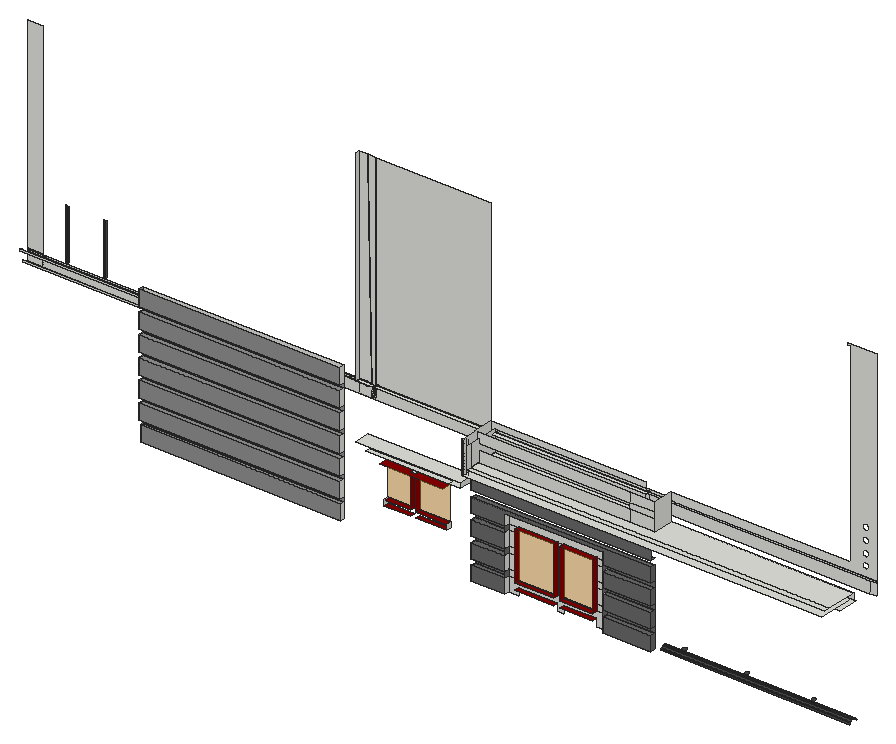
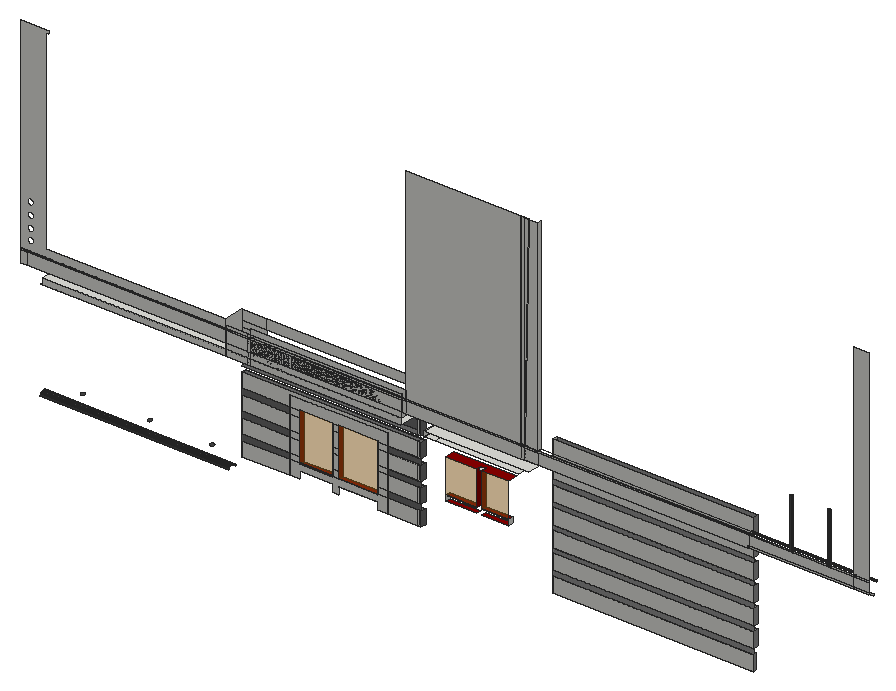
# SketchUp Ruby script. Lengths in inches.
U = 1.inch
M = Sketchup.active_model
def pt(a) = Geom::Point3d.new(a.map { |v| v * U })
def face(e, loops, mat)
  f = e.add_face(loops[0].map { |a| pt(a) })
  loops[1..].each { |l| e.add_face(l.map { |a| pt(a) }).erase! }
  f.material = f.back_material = mat if mat
  f
end
# faces: each face lists its corners as indices into pts; further lists are holes
def faces(e, pts, list, mat = nil) = list.each { |f| face(e, (f[0].is_a?(Array) ? f : [f]).map { |l| l.map { |i| pts[i] } }, mat) }
# xy, xz, yz: faces in a plane at the given z, y or x. An outline is a flat list of corners, or four numbers for a rectangle; further outlines are holes
def ring(l) = l.size == 4 ? [[l[0], l[1]], [l[2], l[1]], [l[2], l[3]], [l[0], l[3]]] : l.each_slice(2).to_a
def flat(e, list, mat, &to3) = list.each { |f| face(e, (f[0].is_a?(Array) ? f : [f]).map { |l| ring(l).map { |u, v| to3.(u, v) } }, mat) }
def xy(e, z, list, mat = nil) = flat(e, list, mat) { |x, y| [x, y, z] }
def xz(e, y, list, mat = nil) = flat(e, list, mat) { |x, z| [x, y, z] }
def yz(e, x, list, mat = nil) = flat(e, list, mat) { |y, z| [x, y, z] }
def lines(e, pts, list) = list.each { |a, b| e.add_line(pt(pts[a]), pt(pts[b])) }
# prism: a flat outline (further loops are holes) pulled along v
def prism(e, loops, v, mat = nil)
  f = face(e, loops, mat); d = Geom::Vector3d.new(v.map { |x| x * U })
  f.pushpull(f.normal.samedirection?(d) ? d.length : -d.length)
end
def box(e, o, s, mat = nil) = prism(e, [[o, [o[0] + s[0], o[1], o[2]], [o[0] + s[0], o[1] + s[1], o[2]], [o[0], o[1] + s[1], o[2]]]], [0, 0, s[2]], mat)
def at(x, y, z, deg = 0) = Geom::Transformation.translation(pt([x, y, z])) * Geom::Transformation.rotation(ORIGIN, Z_AXIS, deg.degrees)
def axes(o, x, y, z) = Geom::Transformation.new([*x, 0, *y, 0, *z, 0, *pt(o).to_a, 1])
def part(name) = M.definitions.add(name)
# library, detail: a bought-in or finely detailed component or shape, given as its bounding box
def library(name, o, s) = part(name).tap { |d| box(d.entities, o, s) }
def detail(e, o, s) = box(e.add_group.entities, o, s)
def put(e, d, t, mat = nil) = e.add_instance(d, t).tap { |i| i.material = mat if mat }
def group(e, t, mat = nil) = e.add_group.tap { |g| g.transformation = t; g.material = mat if mat }.entities
root = M.entities
M.materials.add("[0021_DarkRed]").color = [139, 0, 0]
M.materials.add("[0134_DimGray]").color = [105, 105, 105]
M.materials.add("[0137_Black]").color = [71, 71, 71]
M.materials.add("[Color M05]").color = [145, 145, 145]
M.materials.add("[Translucent Glass Gray]").color = [191, 123, 24]
M.materials["[Translucent Glass Gray]"].alpha = 0.5
xy(root,168.55,[[82.85,16.375,200.79,18.1875]])
xy(root,170.27,[[284.66,7.0625,304.13,10.0625],[362.13,7.0625,390.0625,10.0625]],"[0134_DimGray]")
xy(root,173.53,[[404.27,13.19,404.56,13.23,404.83,13.34,405.0625,13.52,405.24,13.76,405.35,14.03,405.39,14.32,405.35,14.61,405.24,14.88,405.0625,15.11,404.83,15.29,404.56,15.41,404.27,15.44,403.97,15.41,403.7,15.29,403.47,15.11,403.29,14.88,403.18,14.61,403.14,14.32,403.18,14.03,403.29,13.76,403.47,13.52,403.7,13.34,403.97,13.23],[440.77,13.19,441.06,13.23,441.33,13.34,441.5625,13.52,441.74,13.76,441.85,14.03,441.89,14.32,441.85,14.61,441.74,14.88,441.5625,15.11,441.33,15.29,441.06,15.41,440.77,15.44,440.47,15.41,440.2,15.29,439.97,15.11,439.79,14.88,439.68,14.61,439.64,14.32,439.68,14.03,439.79,13.76,439.97,13.52,440.2,13.34,440.47,13.23],[480.14,13.19,480.43,13.23,480.7,13.34,480.9375,13.52,481.12,13.76,481.23,14.03,481.27,14.32,481.23,14.61,481.12,14.88,480.9375,15.11,480.7,15.29,480.43,15.41,480.14,15.44,479.85,15.41,479.58,15.29,479.35,15.11,479.17,14.88,479.05,14.61,479.02,14.32,479.05,14.03,479.17,13.76,479.35,13.52,479.58,13.34,479.85,13.23]],"[0137_Black]")
xy(root,174.59,[[310.13,7.0625,333.13,10.0625],[336.9,7.0625,356.13,10.0625]],"[0021_DarkRed]")
xy(root,177.65,[[82.85,16.375,200.79,18.1875]],"[Color M05]")
xy(root,178.32,[[310.13,7.0625,333.13,10.0625],[336.9,7.0625,356.13,10.0625]],"[0021_DarkRed]")
xy(root,178.6875,[[284.66,7.0625,304.13,10.0625],[362.13,7.0625,390.0625,10.0625]],"[0134_DimGray]")
xy(root,180.55,[[82.85,15.1875,200.79,18.1875]])
xy(root,182.27,[[284.66,7.0625,304.13,10.0625],[362.13,7.0625,390.0625,10.0625]],"[0134_DimGray]")
xy(root,189.65,[[82.85,15.1875,200.79,18.1875]],"[Color M05]")
xy(root,190.54,[[231.66,9.1875,247.4,12.1875],[250.1,9.1875,268.54,12.1875]],"[0021_DarkRed]")
xy(root,190.6875,[[284.66,7.0625,304.13,10.0625],[362.13,7.0625,390.0625,10.0625]],"[0134_DimGray]")
xy(root,192.55,[[82.85,15.1875,200.79,18.1875]])
xy(root,193.6,[[231.66,9.1875,247.4,12.1875],[250.1,9.1875,268.54,12.1875]],"[0021_DarkRed]")
xy(root,194.27,[[284.66,7.0625,304.13,10.0625],[362.13,7.0625,390.0625,10.0625]],"[0134_DimGray]")
xy(root,201.65,[[82.85,15.1875,200.79,18.1875]],"[Color M05]")
xy(root,202.6875,[[284.66,7.0625,304.13,10.0625],[362.13,7.0625,390.0625,10.0625]],"[0134_DimGray]")
xy(root,204.55,[[82.85,15.1875,200.79,18.1875]])
xy(root,206.27,[[284.66,7.0625,304.13,10.0625],[362.13,7.0625,390.0625,10.0625]],"[0134_DimGray]")
xy(root,206.79,[[310.13,7.0625,333.13,10.0625],[336.9,7.0625,356.13,10.0625]],"[0021_DarkRed]")
xy(root,212.79,[[304.13,7.0625,362.13,10.0625]])
xy(root,213.65,[[82.85,15.1875,200.79,18.1875]],"[Color M05]")
xy(root,213.83,[[247.4,9.1875,250.1,12.1875]])
xy(root,213.83,[[231.66,6.1875,231.66,12.1875,247.4,12.1875,247.4,9.1875,250.1,9.1875,250.1,12.1875,268.54,12.1875,268.54,6.1875]],"[0021_DarkRed]")
xy(root,214.6875,[[284.66,7.0625,286.99,10.0625],[286.99,7.0625,390.0625,10.0625]],"[0134_DimGray]")
xy(root,216.55,[[82.85,15.1875,200.79,18.1875]])
xy(root,218.27,[[284.66,7.0625,390.0625,10.0625]],"[0134_DimGray]")
xy(root,219.83,[[225.66,3.1875,274.54,6.1875],[274.54,3.1875,281.16,12.1875],[281.16,3.1875,281.47,12.1875],[225.66,6.1875,274.54,12.1875]])
xy(root,222.71,[[219.91,3.1875,281.47,12.1875]])
xy(root,225.65,[[82.85,15.1875,200.79,18.1875]],"[Color M05]")
xy(root,226.6875,[[335.53,7.0625,375.29,10.0625],[375.29,7.0625,390.0625,10.0625]])
xy(root,226.6875,[[284.66,7.0625,335.53,10.0625]],"[0134_DimGray]")
xy(root,228.47,[[284.05,1.0625,284.41,1.5],[284.41,1.0625,284.41,10.0625,390.0625,10.0625,390.0625,22.0625,495.71,22.0625,495.71,1.0625],[284.41,10.0625,284.66,13.0625],[286.99,10.0625,334.1,22.0625],[334.1,10.0625,375.29,22.0625],
  [375.29,10.0625,390.0625,22.0625],[495.71,10.0625,498.65,22.0625]])
xy(root,228.55,[[82.85,15.1875,200.79,18.1875]])
xy(root,232.22,[[286.99,1.0625,497.29,4.0625],[286.52,4.0625,286.99,22.0625],[286.99,4.0625,497.29,22.0625]])
xy(root,237.65,[[82.85,15.1875,200.79,18.1875]],"[Color M05]")
xy(root,240.55,[[82.85,15.1875,200.79,18.1875]])
xy(root,243,[[206.66,19.6875,214.3,19.75],[206.66,19.75,214.3,22.0625],[214.3,19.75,216.79,21.8125],[216.79,19.75,284.41,22.0625],[284.41,19.75,376.99,22.0625],
  [214.3,21.8125,216.79,22.0625]])
xz(root,1.5,[[284.05,228.47,284.41,247.33]])
xz(root,7.0625,[[284.66,170.27,304.13,178.6875],[362.13,170.27,390.0625,178.6875],[284.66,182.27,304.13,190.6875],[362.13,182.27,390.0625,190.6875],[284.66,194.27,304.13,202.6875],
  [362.13,194.27,390.0625,202.6875],[284.66,206.27,304.13,206.27,304.13,212.79,362.13,212.79,362.13,206.27,390.0625,206.27,390.0625,214.6875,284.66,214.6875],[284.66,218.27,390.0625,226.6875]],"[0134_DimGray]")
xz(root,10.0625,[[284.66,170.27,286.17,178.6875],[286.17,170.27,286.99,178.6875],[286.99,170.27,304.13,178.6875],[304.13,170.27,310.13,170.27,310.13,174.59,333.13,174.59,333.13,170.27,336.9,170.27,336.9,174.59,356.13,174.59,356.13,170.27,362.13,170.27,362.13,178.6875,356.13,178.6875,356.13,178.32,336.9,178.32,336.9,178.6875,333.13,178.6875,333.13,178.32,310.13,178.32,310.13,178.6875,304.13,178.6875],[362.13,170.27,390.0625,178.6875],
  [336.9,178.32,356.13,178.6875],[304.13,178.6875,310.13,182.27],[333.13,178.6875,336.9,182.27],[356.13,178.6875,362.13,182.27],[284.66,182.27,286.17,190.6875],
  [286.17,182.27,286.99,190.6875],[286.99,182.27,304.13,190.6875],[304.13,182.27,310.13,190.6875],[333.13,182.27,336.9,190.6875],[356.13,182.27,362.13,190.6875],
  [362.13,182.27,390.0625,190.6875],[304.13,190.6875,310.13,194.27],[333.13,190.6875,336.9,194.27],[356.13,190.6875,362.13,194.27],[284.66,194.27,286.17,202.6875],
  [286.17,194.27,286.99,202.6875],[286.99,194.27,304.13,202.6875],[304.13,194.27,310.13,202.6875],[333.13,194.27,336.9,202.6875],[356.13,194.27,362.13,202.6875],
  [362.13,194.27,390.0625,202.6875],[304.13,202.6875,310.13,206.27],[333.13,202.6875,336.9,206.27],[356.13,202.6875,362.13,206.27],[284.66,206.27,286.17,214.6875],
  [286.17,206.27,286.99,214.6875],[286.99,206.27,286.99,214.6875,390.0625,214.6875,390.0625,206.27,362.13,206.27,362.13,212.79,304.13,212.79,304.13,206.27],[304.13,206.27,310.13,206.27,310.13,206.79,333.13,206.79,333.13,206.27,336.9,206.27,336.9,206.79,356.13,206.79,356.13,206.27,362.13,206.27,362.13,212.79,304.13,212.79],[284.66,218.27,286.17,226.6875],[286.17,218.27,286.99,226.6875],
  [375.29,228.47,390.0625,230.27],[286.17,230.27,375.29,238.6875],[375.29,230.27,390.0625,238.6875],[375.29,238.6875,390.0625,242.27],[286.17,242.27,375.29,247.89],
  [375.29,242.27,390.0625,247.89]])
xz(root,10.0625,[[284.66,178.6875,304.13,182.27],[362.13,178.6875,390.0625,182.27],[284.66,190.6875,304.13,194.27],[362.13,190.6875,390.0625,194.27],[284.66,202.6875,304.13,206.27],
  [362.13,202.6875,390.0625,206.27]],"[0134_DimGray]")
xz(root,10.0625,[[310.13,178.32,333.13,206.79],[336.9,178.6875,356.13,206.79]],"[Translucent Glass Gray]")
xz(root,12.1875,[[231.66,193.6,247.4,213.83],[250.1,193.6,268.54,213.83]],"[Translucent Glass Gray]")
xz(root,15.1875,[[82.85,180.55,200.79,189.65],[82.85,192.55,200.79,201.65],[82.85,204.55,200.79,213.65],[82.85,216.55,200.79,225.65],[82.85,228.55,200.79,237.65],
  [82.85,240.55,200.79,249.65]],"[Color M05]")
xz(root,16.375,[[82.85,168.55,200.79,177.65]],"[Color M05]")
xz(root,18.1875,[[82.85,168.55,200.79,177.65],[82.85,180.55,200.79,189.65],[82.85,192.55,200.79,201.65],[82.85,204.55,200.79,213.65],[82.85,216.55,200.79,225.65],
  [82.85,228.55,200.79,237.65],[82.85,240.55,200.79,249.65]])
xz(root,18.1875,[[82.85,177.65,200.79,180.55],[82.85,189.65,200.79,192.55],[82.85,201.65,200.79,204.55],[82.85,213.65,200.79,216.55],[82.85,225.65,200.79,228.55],
  [82.85,237.65,200.79,240.55]],"[Color M05]")
xz(root,19.6875,[[9.5625,242.08,82.85,243],[9.5625,243,82.85,243.17]])
xz(root,21.375,[[9.5625,235.42,82.9375,236.47]])
xz(root,21.8125,[[214.3,243,216.79,243,216.79,363,211.87,363]])
xz(root,22.0625,[[286.99,228.47,375.29,228.47,375.29,242.04,286.52,242.04,286.52,232.22,286.99,232.22],[286.99,228.47,375.29,232.22],[375.29,228.47,376.99,232.22],[376.99,228.47,390.0625,232.22],[390.0625,228.47,497.29,232.22],
  [286.52,232.22,375.29,235.42],[375.29,232.22,376.99,235.42],[376.99,232.22,390.0625,235.42],[11.875,235.42,20.875,236.47],[20.875,235.42,82.85,236.47],
  [82.85,235.42,82.9375,236.47],[82.9375,235.42,206.66,235.42,206.66,242.04,82.85,242.04,82.85,236.47,82.9375,236.47],[206.66,235.42,214.43,235.42,214.43,236.48,214.32,242.04,206.66,242.04],[206.66,235.42,216.73,235.42,216.73,242.04,214.32,242.04,214.3,243,214.3,242.04,206.66,242.04],[214.43,235.42,216.73,242.04],
  [216.73,235.42,216.79,242.04],[216.79,235.42,284.41,242.04],[284.41,235.42,286.52,242.04],[286.52,235.42,375.29,242.04],[375.29,235.42,376.99,242.04],
  [376.99,235.42,390.0625,242.04],[390.0625,235.42,507.04,242.04],[507.04,235.42,510.6875,242.04],[11.875,236.47,20.875,242.04],[20.875,236.47,82.85,242.04],
  [214.43,236.48,214.43,242.04,214.32,242.04],[11.875,242.04,20.875,242.08],[20.875,242.04,82.85,242.08],[82.85,242.04,206.66,243],[206.66,242.04,214.29,243],
  [214.29,242.04,214.3,243],[214.3,242.04,214.32,242.04,214.3,243],[214.32,242.04,214.43,242.04,214.43,243,214.3,243],[214.43,242.04,216.73,243],[216.73,242.04,216.79,243],
  [216.79,242.04,284.41,243],[284.41,242.04,286.52,243],[286.52,242.04,375.29,243],[375.29,242.04,376.99,243],[376.99,242.04,390.0625,243],
  [390.0625,242.04,507.04,243],[507.04,242.04,510.6875,243],[11.875,242.08,20.875,243],[20.875,242.08,82.85,243],[11.875,243,20.875,243.17],
  [82.85,243,206.66,243.17],[206.66,243,214.29,243.17],[214.29,243,214.3,243,214.29,243.17],[214.3,243,214.3,243.17,214.29,243.17],[214.3,243,214.43,243.17],
  [214.43,243,216.79,243.17],[216.79,243,284.41,243.17],[284.41,243,286.52,243.17],[286.52,243,375.29,243.17],[375.29,243,376.99,243.17],
  [376.99,243,390.0625,243.17],[390.0625,243,507.04,243.17],[507.04,243,510.6875,243.17],[11.875,243.17,20.6875,363.17],[206.66,243.17,214.29,243.17,211.87,363,206.66,363],
  [214.29,243.17,214.3,243.17,214.3,363,211.87,363],[214.3,243.17,216.79,363],[216.79,243.17,284.41,363],[284.41,243.17,286.52,243.17,286.52,244.84,375.29,244.84,375.29,247.89,284.41,247.89],[286.52,243.17,375.29,244.84],
  [375.29,243.17,376.99,244.84],[376.99,243.17,390.0625,244.84],[[390.0625,243.17,390.0625,247.89,495.71,247.89,495.71,361.6875,494.09,361.6875,494.09,363,510.6875,363,510.6875,243.17],[504.58,260.58,505.05,260.64,505.49,260.83,505.86,261.11,506.15,261.49,506.33,261.93,506.39,262.39,506.33,262.86,506.15,263.3,505.86,263.68,505.49,263.96,505.05,264.15,504.58,264.21,504.11,264.15,503.67,263.96,503.3,263.68,503.01,263.3,502.83,262.86,502.77,262.39,502.83,261.93,503.01,261.49,503.3,261.11,503.67,260.83,504.11,260.64],[504.58,267.58,505.05,267.64,505.49,267.83,505.86,268.11,506.15,268.49,506.33,268.93,506.39,269.39,506.33,269.86,506.15,270.3,505.86,270.68,505.49,270.96,505.05,271.15,504.58,271.21,504.11,271.15,503.67,270.96,503.3,270.68,503.01,270.3,502.83,269.86,502.77,269.39,502.83,268.93,503.01,268.49,503.3,268.11,503.67,267.83,504.11,267.64],[504.58,247.21,505.05,247.27,505.49,247.45,505.86,247.74,506.15,248.11,506.33,248.55,506.39,249.02,506.33,249.49,506.15,249.93,505.86,250.3,505.49,250.59,505.05,250.77,504.58,250.83,504.11,250.77,503.67,250.59,503.3,250.3,503.01,249.93,502.83,249.49,502.77,249.02,502.83,248.55,503.01,248.11,503.3,247.74,503.67,247.45,504.11,247.27],[504.58,253.58,505.05,253.64,505.49,253.83,505.86,254.11,506.15,254.49,506.33,254.93,506.39,255.39,506.33,255.86,506.15,256.3,505.86,256.68,505.49,256.96,505.05,257.15,504.58,257.21,504.11,257.15,503.67,256.96,503.3,256.68,503.01,256.3,502.83,255.86,502.77,255.39,502.83,254.93,503.01,254.49,503.3,254.11,503.67,253.83,504.11,253.64]]])
yz(root,82.85,[[19.6875,242.08,22.0625,243],[19.6875,243,19.75,243.17],[19.75,243,22.0625,243.17]])
yz(root,82.85,[[16.375,168.55,18.1875,177.65],[15.1875,180.55,18.1875,189.65],[15.1875,192.55,18.1875,201.65],[15.1875,204.55,18.1875,213.65],[15.1875,216.55,18.1875,225.65],
  [15.1875,228.55,18.1875,237.65],[15.1875,240.55,18.1875,249.65]],"[Color M05]")
yz(root,82.9375,[[21.375,235.42,22.0625,236.47]])
yz(root,200.79,[[16.375,168.55,18.1875,177.65],[15.1875,180.55,18.1875,189.65],[15.1875,192.55,18.1875,201.65],[15.1875,204.55,18.1875,213.65],[15.1875,216.55,18.1875,225.65],
  [15.1875,228.55,18.1875,237.65],[15.1875,240.55,18.1875,249.65]])
yz(root,206.66,[[19.6875,243,22.0625,363]])
yz(root,216.79,[[21.8125,243,22.0625,363]])
yz(root,231.66,[[9.1875,190.54,12.1875,193.6]])
yz(root,247.4,[[9.1875,193.6,12.1875,213.83]],"[0021_DarkRed]")
yz(root,250.1,[[9.1875,193.6,12.1875,213.83]],"[0021_DarkRed]")
yz(root,268.54,[[9.1875,190.54,12.1875,193.6]])
yz(root,281.47,[[3.1875,219.83,12.1875,222.71]])
yz(root,284.05,[[1.0625,228.47,1.5,247.58]])
yz(root,284.41,[[1.5,228.47,1.5625,247.33],[1.5625,228.47,1.5625,247.33,10.0625,247.33,10.0625,247.89,22.0625,247.89,22.0625,243,13.0625,243,13.0625,228.47]])
yz(root,284.66,[[7.0625,170.27,10.0625,178.6875],[7.0625,182.27,10.0625,190.6875],[7.0625,194.27,10.0625,202.6875],[7.0625,206.27,10.0625,214.6875],[7.0625,218.27,10.0625,226.6875]],"[0134_DimGray]")
yz(root,286.52,[[4.0625,232.22,22.0625,244.84]])
yz(root,286.99,[[1.0625,232.22,4.0625,244.84]])
yz(root,304.13,[[7.0625,170.27,10.0625,178.6875],[7.0625,182.27,10.0625,190.6875],[7.0625,194.27,10.0625,202.6875],[7.0625,206.27,10.0625,212.79]])
yz(root,304.13,[[7.0625,178.6875,10.0625,182.27],[7.0625,190.6875,10.0625,194.27],[7.0625,202.6875,10.0625,206.27]],"[0134_DimGray]")
yz(root,310.13,[[7.0625,178.32,10.0625,206.79]],"[0021_DarkRed]")
yz(root,333.13,[[7.0625,178.32,10.0625,206.79]],"[0021_DarkRed]")
yz(root,336.9,[[7.0625,178.32,10.0625,206.79]],"[0021_DarkRed]")
yz(root,356.13,[[7.0625,178.32,10.0625,206.79]],"[0021_DarkRed]")
yz(root,362.13,[[7.0625,170.27,10.0625,178.6875],[7.0625,182.27,10.0625,190.6875],[7.0625,194.27,10.0625,202.6875],[7.0625,206.27,10.0625,212.79]])
yz(root,362.13,[[7.0625,178.6875,10.0625,182.27],[7.0625,190.6875,10.0625,194.27],[7.0625,202.6875,10.0625,206.27]],"[0134_DimGray]")
yz(root,390.0625,[[10.0625,228.47,22.0625,247.89]])
yz(root,390.0625,[[7.0625,170.27,10.0625,178.6875],[7.0625,182.27,10.0625,190.6875],[7.0625,194.27,10.0625,202.6875],[7.0625,206.27,10.0625,214.6875]],"[0134_DimGray]")
p = [[390.0625,14.85,168.28],[390.0625,14.58,167.65],[501.0625,14.58,167.65],[501.0625,14.85,168.28],[390.0625,19.65,167.65],[390.0625,19.39,168.28],
  [501.0625,19.39,168.28],[501.0625,19.65,167.65],[390.0625,15.26,168.83],[501.0625,15.26,168.83],[390.0625,18.97,168.83],[501.0625,18.97,168.83],
  [390.0625,15.81,169.24],[501.0625,15.81,169.24],[390.0625,18.43,169.24],[501.0625,18.43,169.24],[390.0625,16.4375,169.5],[501.0625,16.4375,169.5],
  [390.0625,17.8,169.5],[501.0625,17.8,169.5],[390.0625,17.12,169.59],[501.0625,17.12,169.59],[214.29,22.0625,243.17],[211.87,22.0625,363],
  [211.87,21.8125,363],[214.3,21.8125,243],[214.3,22.0625,243],[33.8,22.82,243.17],[34.09,22.71,243.17],[34.09,22.71,272.92],
  [33.8,22.82,272.92],[34.4,22.66,243.17],[34.4,22.66,272.92],[34.7,22.71,243.17],[34.7,22.71,272.92],[34.99,22.82,243.17],
  [34.99,22.82,272.92],[33.56,23.01,243.17],[33.56,23.01,272.92],[35.24,23.01,243.17],[35.24,23.01,272.92],[33.37,23.26,243.17],
  [33.37,23.26,272.92],[35.43,23.26,243.17],[35.43,23.26,272.92],[56.16,23.09,243.17],[56.47,23.05,243.17],[56.47,23.05,272.92],
  [56.16,23.09,272.92],[56.78,23.09,243.17],[56.78,23.09,272.92],[55.875,23.21,243.17],[55.875,23.21,272.92],[57.0625,23.21,243.17],
  [57.0625,23.21,272.92],[55.63,23.39,243.17],[55.63,23.39,272.92],[57.31,23.39,243.17],[57.31,23.39,272.92],[33.25,23.54,243.17],
  [33.25,23.54,272.92],[82.85,19.75,243],[206.66,19.75,243],[286.52,1.0625,232.22],[286.52,4.0625,232.22],[285.29,2.8125,247.64],
  [285.29,2.8125,228.47],[286.17,2.8125,247.64],[286.17,2.8125,228.47]]
faces(root,p,[[0,1,2,3],[4,5,6,7],[8,0,3,9],[5,10,11,6],[12,8,9,13],[10,14,15,11],[16,12,13,17],[14,18,19,15],
  [20,16,17,21],[18,20,21,19],[27,28,29,30],[28,31,32,29],[31,33,34,32],[33,35,36,34],[37,27,30,38],[35,39,40,36],
  [41,37,38,42],[39,43,44,40],[45,46,47,48],[46,49,50,47],[51,45,48,52],[49,53,54,50],[55,51,52,56],[53,57,58,54],
  [59,41,42,60]],"[0137_Black]")
faces(root,p,[[22,23,24,25,26]])
lines(root,p,[[61,62],[63,64],[65,66],[67,68]])
